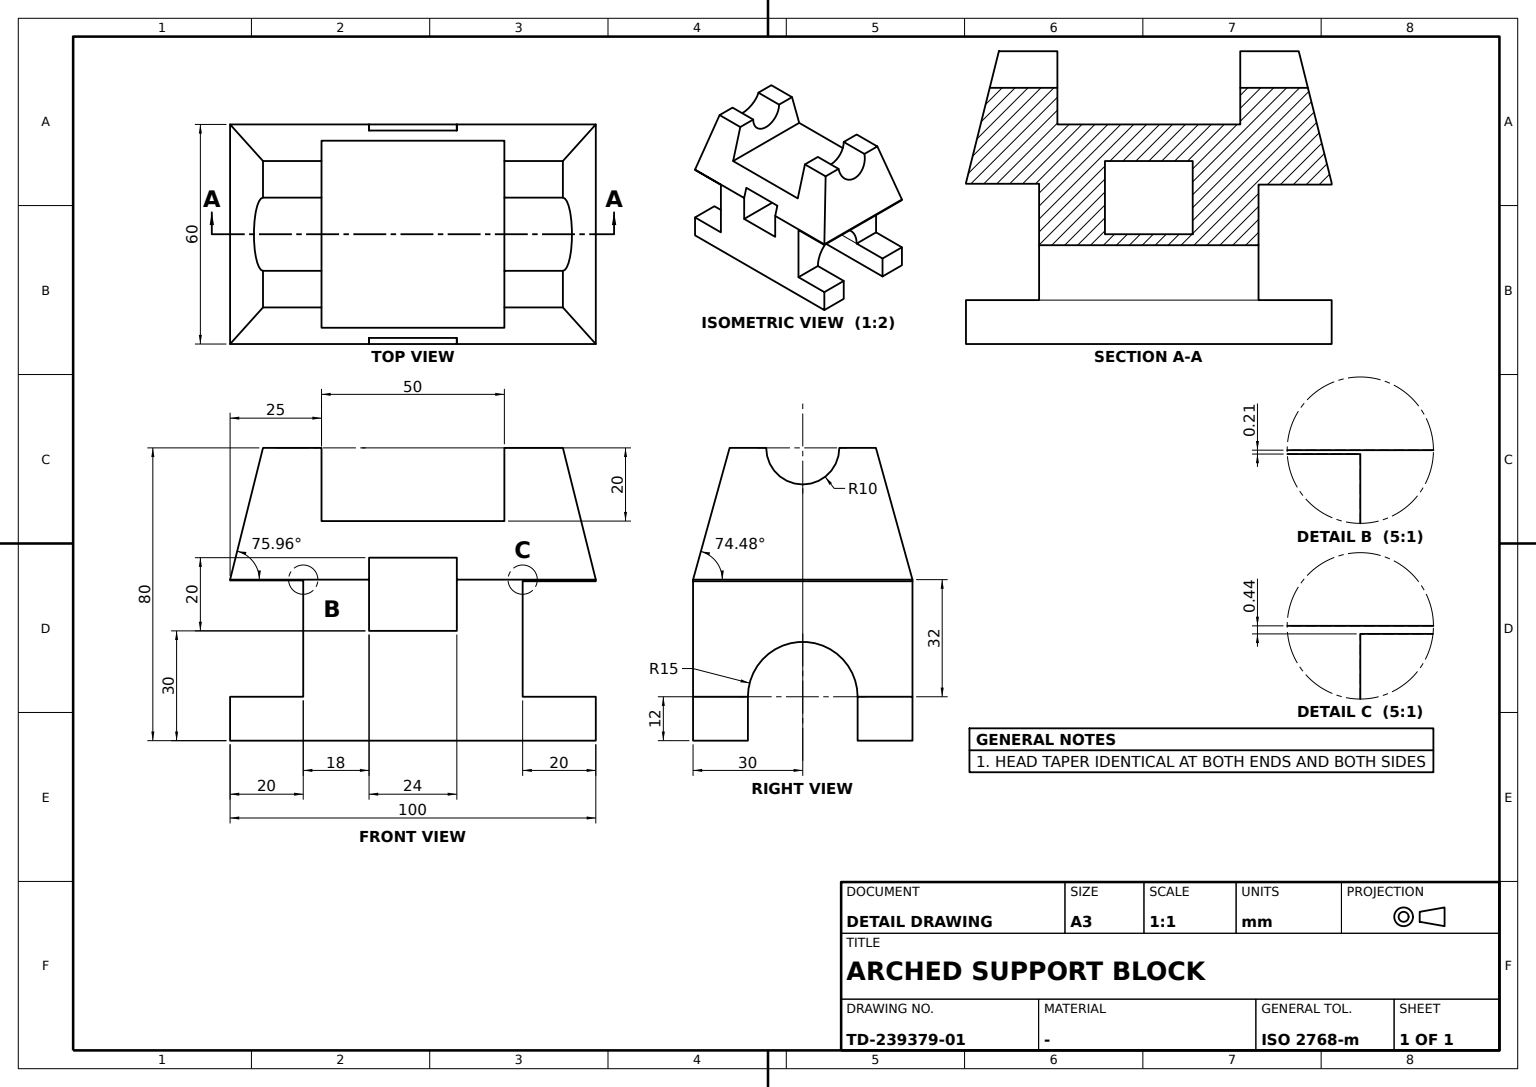
ISO-10303-21;
HEADER;
FILE_DESCRIPTION((''),'2;1');
FILE_NAME('','',(''),(''),'','','');
FILE_SCHEMA(('AUTOMOTIVE_DESIGN'));
ENDSEC;
DATA;
#1=APPLICATION_CONTEXT('');
#2=PRODUCT_CONTEXT('',#1,'mechanical');
#3=PRODUCT('','','',(#2));
#4=PRODUCT_DEFINITION_FORMATION('','',#3);
#5=PRODUCT_DEFINITION_CONTEXT('',#1,'design');
#6=PRODUCT_DEFINITION('','',#4,#5);
#7=PRODUCT_DEFINITION_SHAPE('','',#6);
#8=(LENGTH_UNIT()NAMED_UNIT(*)SI_UNIT(.MILLI.,.METRE.));
#9=(NAMED_UNIT(*)PLANE_ANGLE_UNIT()SI_UNIT($,.RADIAN.));
#10=(NAMED_UNIT(*)SI_UNIT($,.STERADIAN.)SOLID_ANGLE_UNIT());
#11=UNCERTAINTY_MEASURE_WITH_UNIT(LENGTH_MEASURE(0.005),#8,'distance_accuracy_value','');
#12=(GEOMETRIC_REPRESENTATION_CONTEXT(3)GLOBAL_UNCERTAINTY_ASSIGNED_CONTEXT((#11))GLOBAL_UNIT_ASSIGNED_CONTEXT((#8,#9,#10))REPRESENTATION_CONTEXT('',''));
#13=CARTESIAN_POINT('',(40.,25.,80.));
#14=VERTEX_POINT('',#13);
#15=CARTESIAN_POINT('',(20.,25.,80.));
#16=VERTEX_POINT('',#15);
#17=CARTESIAN_POINT('',(30.,25.,80.));
#18=DIRECTION('',(0.,1.,0.));
#19=DIRECTION('',(0.,0.,1.));
#20=AXIS2_PLACEMENT_3D('',#17,#18,#19);
#21=CIRCLE('',#20,10.);
#22=EDGE_CURVE('',#14,#16,#21,.T.);
#23=ORIENTED_EDGE('',*,*,#22,.T.);
#24=CARTESIAN_POINT('',(20.,9.,80.));
#25=VERTEX_POINT('',#24);
#26=VECTOR('',#18,1000.);
#27=LINE('',#24,#26);
#28=EDGE_CURVE('',#25,#16,#27,.T.);
#29=ORIENTED_EDGE('',*,*,#28,.F.);
#30=CARTESIAN_POINT('',(40.,9.,80.));
#31=VERTEX_POINT('',#30);
#32=CARTESIAN_POINT('',(30.,9.,80.));
#33=DIRECTION('',(0.,-0.9701425,0.242535625));
#34=DIRECTION('',(0.,0.242535625,0.9701425));
#35=AXIS2_PLACEMENT_3D('',#32,#33,#34);
#36=ELLIPSE('',#35,10.307764,10.);
#37=EDGE_CURVE('',#25,#31,#36,.T.);
#38=ORIENTED_EDGE('',*,*,#37,.T.);
#39=LINE('',#30,#26);
#40=EDGE_CURVE('',#14,#31,#39,.F.);
#41=ORIENTED_EDGE('',*,*,#40,.F.);
#42=EDGE_LOOP('',(#23,#29,#38,#41));
#43=FACE_BOUND('',#42,.T.);
#44=CARTESIAN_POINT('',(30.,49.34,80.));
#45=DIRECTION('',(-1.,0.,0.));
#46=AXIS2_PLACEMENT_3D('',#44,#18,#45);
#47=CYLINDRICAL_SURFACE('',#46,10.);
#48=ADVANCED_FACE('',(#43),#47,.F.);
#49=CARTESIAN_POINT('',(60.,100.,0.));
#50=VERTEX_POINT('',#49);
#51=CARTESIAN_POINT('',(60.,100.,12.));
#52=VERTEX_POINT('',#51);
#53=VECTOR('',#19,1000.);
#54=LINE('',#49,#53);
#55=EDGE_CURVE('',#50,#52,#54,.T.);
#56=ORIENTED_EDGE('',*,*,#55,.F.);
#57=CARTESIAN_POINT('',(45.,100.,0.));
#58=VERTEX_POINT('',#57);
#59=CARTESIAN_POINT('',(0.,100.,0.));
#60=VECTOR('',#45,1000.);
#61=LINE('',#59,#60);
#62=EDGE_CURVE('',#50,#58,#61,.T.);
#63=ORIENTED_EDGE('',*,*,#62,.T.);
#64=CARTESIAN_POINT('',(45.,100.,12.));
#65=VERTEX_POINT('',#64);
#66=DIRECTION('',(0.,0.,-1.));
#67=VECTOR('',#66,1000.);
#68=LINE('',#64,#67);
#69=EDGE_CURVE('',#65,#58,#68,.T.);
#70=ORIENTED_EDGE('',*,*,#69,.F.);
#71=CARTESIAN_POINT('',(15.,100.,12.));
#72=LINE('',#71,#60);
#73=EDGE_CURVE('',#52,#65,#72,.T.);
#74=ORIENTED_EDGE('',*,*,#73,.F.);
#75=EDGE_LOOP('',(#56,#63,#70,#74));
#76=FACE_BOUND('',#75,.T.);
#77=AXIS2_PLACEMENT_3D('',#49,#18,#45);
#78=PLANE('',#77);
#79=ADVANCED_FACE('',(#76),#78,.T.);
#80=CARTESIAN_POINT('',(60.,0.,0.));
#81=VERTEX_POINT('',#80);
#82=CARTESIAN_POINT('',(60.,0.,12.));
#83=VERTEX_POINT('',#82);
#84=LINE('',#80,#53);
#85=EDGE_CURVE('',#81,#83,#84,.T.);
#86=ORIENTED_EDGE('',*,*,#85,.T.);
#87=CARTESIAN_POINT('',(45.,0.,12.));
#88=VERTEX_POINT('',#87);
#89=CARTESIAN_POINT('',(15.,0.,12.));
#90=DIRECTION('',(1.,0.,0.));
#91=VECTOR('',#90,1000.);
#92=LINE('',#89,#91);
#93=EDGE_CURVE('',#88,#83,#92,.T.);
#94=ORIENTED_EDGE('',*,*,#93,.F.);
#95=CARTESIAN_POINT('',(45.,0.,0.));
#96=VERTEX_POINT('',#95);
#97=LINE('',#95,#67);
#98=EDGE_CURVE('',#88,#96,#97,.T.);
#99=ORIENTED_EDGE('',*,*,#98,.T.);
#100=CARTESIAN_POINT('',(0.,0.,0.));
#101=LINE('',#100,#91);
#102=EDGE_CURVE('',#96,#81,#101,.T.);
#103=ORIENTED_EDGE('',*,*,#102,.T.);
#104=EDGE_LOOP('',(#86,#94,#99,#103));
#105=FACE_BOUND('',#104,.T.);
#106=DIRECTION('',(0.,-1.,0.));
#107=AXIS2_PLACEMENT_3D('',#100,#106,#90);
#108=PLANE('',#107);
#109=ADVANCED_FACE('',(#105),#108,.T.);
#110=CARTESIAN_POINT('',(15.,80.,12.));
#111=VERTEX_POINT('',#110);
#112=CARTESIAN_POINT('',(0.,80.,12.));
#113=VERTEX_POINT('',#112);
#114=LINE('',#110,#60);
#115=EDGE_CURVE('',#111,#113,#114,.T.);
#116=ORIENTED_EDGE('',*,*,#115,.T.);
#117=CARTESIAN_POINT('',(0.,80.,43.56));
#118=VERTEX_POINT('',#117);
#119=CARTESIAN_POINT('',(0.,80.,0.));
#120=LINE('',#119,#53);
#121=EDGE_CURVE('',#113,#118,#120,.T.);
#122=ORIENTED_EDGE('',*,*,#121,.T.);
#123=CARTESIAN_POINT('',(60.,80.,43.56));
#124=VERTEX_POINT('',#123);
#125=LINE('',#117,#91);
#126=EDGE_CURVE('',#118,#124,#125,.T.);
#127=ORIENTED_EDGE('',*,*,#126,.T.);
#128=CARTESIAN_POINT('',(60.,80.,12.));
#129=VERTEX_POINT('',#128);
#130=CARTESIAN_POINT('',(60.,80.,0.));
#131=LINE('',#130,#67);
#132=EDGE_CURVE('',#124,#129,#131,.T.);
#133=ORIENTED_EDGE('',*,*,#132,.T.);
#134=CARTESIAN_POINT('',(45.,80.,12.));
#135=VERTEX_POINT('',#134);
#136=EDGE_CURVE('',#129,#135,#114,.T.);
#137=ORIENTED_EDGE('',*,*,#136,.T.);
#138=CARTESIAN_POINT('',(30.,80.,12.));
#139=AXIS2_PLACEMENT_3D('',#138,#18,#19);
#140=CIRCLE('',#139,15.);
#141=EDGE_CURVE('',#111,#135,#140,.T.);
#142=ORIENTED_EDGE('',*,*,#141,.F.);
#143=EDGE_LOOP('',(#116,#122,#127,#133,#137,#142));
#144=FACE_BOUND('',#143,.T.);
#145=AXIS2_PLACEMENT_3D('',#119,#18,#45);
#146=PLANE('',#145);
#147=ADVANCED_FACE('',(#144),#146,.T.);
#148=CARTESIAN_POINT('',(1.666667,38.,50.));
#149=VERTEX_POINT('',#148);
#150=CARTESIAN_POINT('',(58.333333,38.,50.));
#151=VERTEX_POINT('',#150);
#152=CARTESIAN_POINT('',(0.,38.,50.));
#153=LINE('',#152,#91);
#154=EDGE_CURVE('',#149,#151,#153,.T.);
#155=ORIENTED_EDGE('',*,*,#154,.T.);
#156=CARTESIAN_POINT('',(60.,38.,44.));
#157=VERTEX_POINT('',#156);
#158=CARTESIAN_POINT('',(59.312321,38.,46.475645));
#159=DIRECTION('',(0.267643864,0.,-0.96351791));
#160=VECTOR('',#159,1000.);
#161=LINE('',#158,#160);
#162=EDGE_CURVE('',#151,#157,#161,.T.);
#163=ORIENTED_EDGE('',*,*,#162,.T.);
#164=CARTESIAN_POINT('',(60.,38.,30.));
#165=VERTEX_POINT('',#164);
#166=LINE('',#164,#53);
#167=EDGE_CURVE('',#165,#157,#166,.T.);
#168=ORIENTED_EDGE('',*,*,#167,.F.);
#169=CARTESIAN_POINT('',(0.,38.,30.));
#170=VERTEX_POINT('',#169);
#171=LINE('',#169,#91);
#172=EDGE_CURVE('',#170,#165,#171,.T.);
#173=ORIENTED_EDGE('',*,*,#172,.F.);
#174=CARTESIAN_POINT('',(0.,38.,44.));
#175=VERTEX_POINT('',#174);
#176=CARTESIAN_POINT('',(0.,38.,0.));
#177=LINE('',#176,#53);
#178=EDGE_CURVE('',#170,#175,#177,.T.);
#179=ORIENTED_EDGE('',*,*,#178,.T.);
#180=DIRECTION('',(0.267643864,0.,0.96351791));
#181=VECTOR('',#180,1000.);
#182=LINE('',#174,#181);
#183=EDGE_CURVE('',#175,#149,#182,.T.);
#184=ORIENTED_EDGE('',*,*,#183,.T.);
#185=EDGE_LOOP('',(#155,#163,#168,#173,#179,#184));
#186=FACE_BOUND('',#185,.T.);
#187=AXIS2_PLACEMENT_3D('',#169,#18,#19);
#188=PLANE('',#187);
#189=ADVANCED_FACE('',(#186),#188,.T.);
#190=VERTEX_POINT('',#100);
#191=CARTESIAN_POINT('',(0.,0.,12.));
#192=VERTEX_POINT('',#191);
#193=LINE('',#100,#53);
#194=EDGE_CURVE('',#190,#192,#193,.T.);
#195=ORIENTED_EDGE('',*,*,#194,.F.);
#196=CARTESIAN_POINT('',(15.,0.,0.));
#197=VERTEX_POINT('',#196);
#198=EDGE_CURVE('',#190,#197,#101,.T.);
#199=ORIENTED_EDGE('',*,*,#198,.T.);
#200=VERTEX_POINT('',#89);
#201=LINE('',#196,#53);
#202=EDGE_CURVE('',#197,#200,#201,.T.);
#203=ORIENTED_EDGE('',*,*,#202,.T.);
#204=EDGE_CURVE('',#192,#200,#92,.T.);
#205=ORIENTED_EDGE('',*,*,#204,.F.);
#206=EDGE_LOOP('',(#195,#199,#203,#205));
#207=FACE_BOUND('',#206,.T.);
#208=ADVANCED_FACE('',(#207),#108,.T.);
#209=CARTESIAN_POINT('',(0.,62.,30.));
#210=VERTEX_POINT('',#209);
#211=CARTESIAN_POINT('',(60.,62.,30.));
#212=VERTEX_POINT('',#211);
#213=LINE('',#209,#91);
#214=EDGE_CURVE('',#210,#212,#213,.T.);
#215=ORIENTED_EDGE('',*,*,#214,.F.);
#216=CARTESIAN_POINT('',(0.,0.,30.));
#217=LINE('',#216,#26);
#218=EDGE_CURVE('',#170,#210,#217,.T.);
#219=ORIENTED_EDGE('',*,*,#218,.F.);
#220=ORIENTED_EDGE('',*,*,#172,.T.);
#221=LINE('',#164,#26);
#222=EDGE_CURVE('',#165,#212,#221,.T.);
#223=ORIENTED_EDGE('',*,*,#222,.T.);
#224=EDGE_LOOP('',(#215,#219,#220,#223));
#225=FACE_BOUND('',#224,.T.);
#226=AXIS2_PLACEMENT_3D('',#169,#66,#18);
#227=PLANE('',#226);
#228=ADVANCED_FACE('',(#225),#227,.F.);
#229=CARTESIAN_POINT('',(40.,91.,80.));
#230=VERTEX_POINT('',#229);
#231=CARTESIAN_POINT('',(50.,91.,80.));
#232=VERTEX_POINT('',#231);
#233=LINE('',#231,#91);
#234=EDGE_CURVE('',#230,#232,#233,.T.);
#235=ORIENTED_EDGE('',*,*,#234,.F.);
#236=CARTESIAN_POINT('',(40.,75.,80.));
#237=VERTEX_POINT('',#236);
#238=LINE('',#236,#26);
#239=EDGE_CURVE('',#230,#237,#238,.F.);
#240=ORIENTED_EDGE('',*,*,#239,.T.);
#241=CARTESIAN_POINT('',(50.,75.,80.));
#242=VERTEX_POINT('',#241);
#243=LINE('',#241,#91);
#244=EDGE_CURVE('',#237,#242,#243,.T.);
#245=ORIENTED_EDGE('',*,*,#244,.T.);
#246=CARTESIAN_POINT('',(50.,100.,80.));
#247=VECTOR('',#106,1000.);
#248=LINE('',#246,#247);
#249=EDGE_CURVE('',#232,#242,#248,.T.);
#250=ORIENTED_EDGE('',*,*,#249,.F.);
#251=EDGE_LOOP('',(#235,#240,#245,#250));
#252=FACE_BOUND('',#251,.T.);
#253=AXIS2_PLACEMENT_3D('',#246,#19,#45);
#254=PLANE('',#253);
#255=ADVANCED_FACE('',(#252),#254,.T.);
#256=CARTESIAN_POINT('',(0.,100.,44.));
#257=VERTEX_POINT('',#256);
#258=CARTESIAN_POINT('',(60.,100.,44.));
#259=VERTEX_POINT('',#258);
#260=LINE('',#256,#91);
#261=EDGE_CURVE('',#257,#259,#260,.T.);
#262=ORIENTED_EDGE('',*,*,#261,.F.);
#263=CARTESIAN_POINT('',(10.,91.,80.));
#264=VERTEX_POINT('',#263);
#265=CARTESIAN_POINT('',(9.322952,91.609343,77.562627));
#266=DIRECTION('',(0.260201474,-0.234181327,0.936725306));
#267=VECTOR('',#266,1000.);
#268=LINE('',#265,#267);
#269=EDGE_CURVE('',#257,#264,#268,.T.);
#270=ORIENTED_EDGE('',*,*,#269,.T.);
#271=CARTESIAN_POINT('',(20.,91.,80.));
#272=VERTEX_POINT('',#271);
#273=EDGE_CURVE('',#264,#272,#233,.T.);
#274=ORIENTED_EDGE('',*,*,#273,.T.);
#275=CARTESIAN_POINT('',(30.,91.,80.));
#276=DIRECTION('',(0.,-0.9701425,-0.242535625));
#277=DIRECTION('',(0.,0.242535625,-0.9701425));
#278=AXIS2_PLACEMENT_3D('',#275,#276,#277);
#279=ELLIPSE('',#278,10.307764,10.);
#280=EDGE_CURVE('',#272,#230,#279,.T.);
#281=ORIENTED_EDGE('',*,*,#280,.T.);
#282=ORIENTED_EDGE('',*,*,#234,.T.);
#283=CARTESIAN_POINT('',(46.61476,87.953284,92.186865));
#284=DIRECTION('',(-0.260201474,-0.234181327,0.936725306));
#285=VECTOR('',#284,1000.);
#286=LINE('',#283,#285);
#287=EDGE_CURVE('',#259,#232,#286,.T.);
#288=ORIENTED_EDGE('',*,*,#287,.F.);
#289=EDGE_LOOP('',(#262,#270,#274,#281,#282,#288));
#290=FACE_BOUND('',#289,.T.);
#291=CARTESIAN_POINT('',(0.,91.,80.));
#292=AXIS2_PLACEMENT_3D('',#291,#276,#277);
#293=PLANE('',#292);
#294=ADVANCED_FACE('',(#290),#293,.F.);
#295=CARTESIAN_POINT('',(50.,25.,80.));
#296=VERTEX_POINT('',#295);
#297=CARTESIAN_POINT('',(55.555556,25.,60.));
#298=VERTEX_POINT('',#297);
#299=CARTESIAN_POINT('',(51.575931,25.,74.326648));
#300=LINE('',#299,#160);
#301=EDGE_CURVE('',#296,#298,#300,.T.);
#302=ORIENTED_EDGE('',*,*,#301,.T.);
#303=CARTESIAN_POINT('',(4.444444,25.,60.));
#304=VERTEX_POINT('',#303);
#305=CARTESIAN_POINT('',(0.,25.,60.));
#306=LINE('',#305,#91);
#307=EDGE_CURVE('',#304,#298,#306,.T.);
#308=ORIENTED_EDGE('',*,*,#307,.F.);
#309=CARTESIAN_POINT('',(10.,25.,80.));
#310=VERTEX_POINT('',#309);
#311=CARTESIAN_POINT('',(4.126074,25.,58.853868));
#312=DIRECTION('',(-0.267643864,0.,-0.96351791));
#313=VECTOR('',#312,1000.);
#314=LINE('',#311,#313);
#315=EDGE_CURVE('',#310,#304,#314,.T.);
#316=ORIENTED_EDGE('',*,*,#315,.F.);
#317=CARTESIAN_POINT('',(0.,25.,80.));
#318=LINE('',#317,#91);
#319=EDGE_CURVE('',#310,#16,#318,.T.);
#320=ORIENTED_EDGE('',*,*,#319,.T.);
#321=ORIENTED_EDGE('',*,*,#22,.F.);
#322=EDGE_CURVE('',#14,#296,#318,.T.);
#323=ORIENTED_EDGE('',*,*,#322,.T.);
#324=EDGE_LOOP('',(#302,#308,#316,#320,#321,#323));
#325=FACE_BOUND('',#324,.T.);
#326=AXIS2_PLACEMENT_3D('',#305,#18,#19);
#327=PLANE('',#326);
#328=ADVANCED_FACE('',(#325),#327,.T.);
#329=CARTESIAN_POINT('',(0.,20.,12.));
#330=VERTEX_POINT('',#329);
#331=CARTESIAN_POINT('',(15.,20.,12.));
#332=VERTEX_POINT('',#331);
#333=LINE('',#331,#91);
#334=EDGE_CURVE('',#330,#332,#333,.T.);
#335=ORIENTED_EDGE('',*,*,#334,.T.);
#336=CARTESIAN_POINT('',(45.,20.,12.));
#337=VERTEX_POINT('',#336);
#338=CARTESIAN_POINT('',(30.,20.,12.));
#339=AXIS2_PLACEMENT_3D('',#338,#106,#66);
#340=CIRCLE('',#339,15.);
#341=EDGE_CURVE('',#337,#332,#340,.T.);
#342=ORIENTED_EDGE('',*,*,#341,.F.);
#343=CARTESIAN_POINT('',(60.,20.,12.));
#344=VERTEX_POINT('',#343);
#345=EDGE_CURVE('',#337,#344,#333,.T.);
#346=ORIENTED_EDGE('',*,*,#345,.T.);
#347=CARTESIAN_POINT('',(60.,20.,43.788128));
#348=VERTEX_POINT('',#347);
#349=CARTESIAN_POINT('',(60.,20.,0.));
#350=LINE('',#349,#53);
#351=EDGE_CURVE('',#344,#348,#350,.T.);
#352=ORIENTED_EDGE('',*,*,#351,.T.);
#353=CARTESIAN_POINT('',(0.,20.,43.788128));
#354=VERTEX_POINT('',#353);
#355=LINE('',#347,#60);
#356=EDGE_CURVE('',#348,#354,#355,.T.);
#357=ORIENTED_EDGE('',*,*,#356,.T.);
#358=CARTESIAN_POINT('',(0.,20.,0.));
#359=LINE('',#358,#67);
#360=EDGE_CURVE('',#354,#330,#359,.T.);
#361=ORIENTED_EDGE('',*,*,#360,.T.);
#362=EDGE_LOOP('',(#335,#342,#346,#352,#357,#361));
#363=FACE_BOUND('',#362,.T.);
#364=AXIS2_PLACEMENT_3D('',#358,#106,#90);
#365=PLANE('',#364);
#366=ADVANCED_FACE('',(#363),#365,.T.);
#367=LINE('',#95,#247);
#368=EDGE_CURVE('',#58,#96,#367,.T.);
#369=ORIENTED_EDGE('',*,*,#368,.T.);
#370=ORIENTED_EDGE('',*,*,#98,.F.);
#371=LINE('',#64,#26);
#372=EDGE_CURVE('',#88,#337,#371,.T.);
#373=ORIENTED_EDGE('',*,*,#372,.T.);
#374=CARTESIAN_POINT('',(45.,50.,12.));
#375=LINE('',#374,#26);
#376=EDGE_CURVE('',#135,#337,#375,.F.);
#377=ORIENTED_EDGE('',*,*,#376,.F.);
#378=LINE('',#64,#247);
#379=EDGE_CURVE('',#65,#135,#378,.T.);
#380=ORIENTED_EDGE('',*,*,#379,.F.);
#381=ORIENTED_EDGE('',*,*,#69,.T.);
#382=EDGE_LOOP('',(#369,#370,#373,#377,#380,#381));
#383=FACE_BOUND('',#382,.T.);
#384=AXIS2_PLACEMENT_3D('',#64,#45,#66);
#385=PLANE('',#384);
#386=ADVANCED_FACE('',(#383),#385,.T.);
#387=CARTESIAN_POINT('',(55.555556,75.,60.));
#388=VERTEX_POINT('',#387);
#389=CARTESIAN_POINT('',(55.555556,100.,60.));
#390=LINE('',#389,#26);
#391=EDGE_CURVE('',#298,#388,#390,.T.);
#392=ORIENTED_EDGE('',*,*,#391,.T.);
#393=CARTESIAN_POINT('',(4.444444,75.,60.));
#394=VERTEX_POINT('',#393);
#395=CARTESIAN_POINT('',(0.,75.,60.));
#396=LINE('',#395,#91);
#397=EDGE_CURVE('',#394,#388,#396,.T.);
#398=ORIENTED_EDGE('',*,*,#397,.F.);
#399=CARTESIAN_POINT('',(4.444444,100.,60.));
#400=LINE('',#399,#26);
#401=EDGE_CURVE('',#304,#394,#400,.T.);
#402=ORIENTED_EDGE('',*,*,#401,.F.);
#403=ORIENTED_EDGE('',*,*,#307,.T.);
#404=EDGE_LOOP('',(#392,#398,#402,#403));
#405=FACE_BOUND('',#404,.T.);
#406=AXIS2_PLACEMENT_3D('',#305,#66,#18);
#407=PLANE('',#406);
#408=ADVANCED_FACE('',(#405),#407,.F.);
#409=ORIENTED_EDGE('',*,*,#368,.F.);
#410=ORIENTED_EDGE('',*,*,#62,.F.);
#411=LINE('',#80,#247);
#412=EDGE_CURVE('',#50,#81,#411,.T.);
#413=ORIENTED_EDGE('',*,*,#412,.T.);
#414=ORIENTED_EDGE('',*,*,#102,.F.);
#415=EDGE_LOOP('',(#409,#410,#413,#414));
#416=FACE_BOUND('',#415,.T.);
#417=AXIS2_PLACEMENT_3D('',#100,#19,#18);
#418=PLANE('',#417);
#419=ADVANCED_FACE('',(#416),#418,.F.);
#420=ORIENTED_EDGE('',*,*,#249,.T.);
#421=CARTESIAN_POINT('',(60.,75.,44.));
#422=LINE('',#421,#160);
#423=EDGE_CURVE('',#242,#388,#422,.T.);
#424=ORIENTED_EDGE('',*,*,#423,.T.);
#425=ORIENTED_EDGE('',*,*,#391,.F.);
#426=ORIENTED_EDGE('',*,*,#301,.F.);
#427=CARTESIAN_POINT('',(50.,9.,80.));
#428=VERTEX_POINT('',#427);
#429=EDGE_CURVE('',#296,#428,#248,.T.);
#430=ORIENTED_EDGE('',*,*,#429,.T.);
#431=CARTESIAN_POINT('',(60.,0.,44.));
#432=VERTEX_POINT('',#431);
#433=CARTESIAN_POINT('',(46.61476,12.046716,92.186865));
#434=DIRECTION('',(-0.260201474,0.234181327,0.936725306));
#435=VECTOR('',#434,1000.);
#436=LINE('',#433,#435);
#437=EDGE_CURVE('',#432,#428,#436,.T.);
#438=ORIENTED_EDGE('',*,*,#437,.F.);
#439=LINE('',#258,#247);
#440=EDGE_CURVE('',#157,#432,#439,.T.);
#441=ORIENTED_EDGE('',*,*,#440,.F.);
#442=ORIENTED_EDGE('',*,*,#162,.F.);
#443=CARTESIAN_POINT('',(58.333333,62.,50.));
#444=VERTEX_POINT('',#443);
#445=CARTESIAN_POINT('',(58.333333,100.,50.));
#446=LINE('',#445,#247);
#447=EDGE_CURVE('',#444,#151,#446,.T.);
#448=ORIENTED_EDGE('',*,*,#447,.F.);
#449=CARTESIAN_POINT('',(60.,62.,44.));
#450=VERTEX_POINT('',#449);
#451=LINE('',#449,#160);
#452=EDGE_CURVE('',#444,#450,#451,.T.);
#453=ORIENTED_EDGE('',*,*,#452,.T.);
#454=EDGE_CURVE('',#259,#450,#439,.T.);
#455=ORIENTED_EDGE('',*,*,#454,.F.);
#456=ORIENTED_EDGE('',*,*,#287,.T.);
#457=EDGE_LOOP('',(#420,#424,#425,#426,#430,#438,#441,#442,#448,#453,#455,#456));
#458=FACE_BOUND('',#457,.T.);
#459=DIRECTION('',(0.96351791,0.,0.267643864));
#460=DIRECTION('',(-0.267643864,0.,0.96351791));
#461=AXIS2_PLACEMENT_3D('',#258,#459,#460);
#462=PLANE('',#461);
#463=ADVANCED_FACE('',(#458),#462,.T.);
#464=ORIENTED_EDGE('',*,*,#204,.T.);
#465=LINE('',#71,#26);
#466=EDGE_CURVE('',#200,#332,#465,.T.);
#467=ORIENTED_EDGE('',*,*,#466,.T.);
#468=ORIENTED_EDGE('',*,*,#334,.F.);
#469=CARTESIAN_POINT('',(0.,100.,12.));
#470=LINE('',#469,#26);
#471=EDGE_CURVE('',#192,#330,#470,.T.);
#472=ORIENTED_EDGE('',*,*,#471,.F.);
#473=EDGE_LOOP('',(#464,#467,#468,#472));
#474=FACE_BOUND('',#473,.T.);
#475=AXIS2_PLACEMENT_3D('',#71,#19,#45);
#476=PLANE('',#475);
#477=ADVANCED_FACE('',(#474),#476,.T.);
#478=CARTESIAN_POINT('',(60.,62.,0.));
#479=LINE('',#478,#53);
#480=EDGE_CURVE('',#212,#450,#479,.T.);
#481=ORIENTED_EDGE('',*,*,#480,.T.);
#482=ORIENTED_EDGE('',*,*,#452,.F.);
#483=CARTESIAN_POINT('',(1.666667,62.,50.));
#484=VERTEX_POINT('',#483);
#485=CARTESIAN_POINT('',(0.,62.,50.));
#486=LINE('',#485,#91);
#487=EDGE_CURVE('',#484,#444,#486,.T.);
#488=ORIENTED_EDGE('',*,*,#487,.F.);
#489=CARTESIAN_POINT('',(0.,62.,44.));
#490=VERTEX_POINT('',#489);
#491=CARTESIAN_POINT('',(1.547278,62.,49.570201));
#492=LINE('',#491,#181);
#493=EDGE_CURVE('',#490,#484,#492,.T.);
#494=ORIENTED_EDGE('',*,*,#493,.F.);
#495=CARTESIAN_POINT('',(0.,62.,0.));
#496=LINE('',#495,#67);
#497=EDGE_CURVE('',#490,#210,#496,.T.);
#498=ORIENTED_EDGE('',*,*,#497,.T.);
#499=ORIENTED_EDGE('',*,*,#214,.T.);
#500=EDGE_LOOP('',(#481,#482,#488,#494,#498,#499));
#501=FACE_BOUND('',#500,.T.);
#502=AXIS2_PLACEMENT_3D('',#485,#106,#66);
#503=PLANE('',#502);
#504=ADVANCED_FACE('',(#501),#503,.T.);
#505=CARTESIAN_POINT('',(15.,50.,12.));
#506=LINE('',#505,#26);
#507=EDGE_CURVE('',#111,#332,#506,.F.);
#508=ORIENTED_EDGE('',*,*,#507,.F.);
#509=ORIENTED_EDGE('',*,*,#141,.T.);
#510=ORIENTED_EDGE('',*,*,#376,.T.);
#511=ORIENTED_EDGE('',*,*,#341,.T.);
#512=EDGE_LOOP('',(#508,#509,#510,#511));
#513=FACE_BOUND('',#512,.T.);
#514=CARTESIAN_POINT('',(30.,50.,12.));
#515=AXIS2_PLACEMENT_3D('',#514,#18,#45);
#516=CYLINDRICAL_SURFACE('',#515,15.);
#517=ADVANCED_FACE('',(#513),#516,.F.);
#518=CARTESIAN_POINT('',(0.,0.,44.));
#519=VERTEX_POINT('',#518);
#520=LINE('',#518,#91);
#521=EDGE_CURVE('',#519,#432,#520,.T.);
#522=ORIENTED_EDGE('',*,*,#521,.T.);
#523=ORIENTED_EDGE('',*,*,#437,.T.);
#524=LINE('',#427,#91);
#525=EDGE_CURVE('',#31,#428,#524,.T.);
#526=ORIENTED_EDGE('',*,*,#525,.F.);
#527=ORIENTED_EDGE('',*,*,#37,.F.);
#528=CARTESIAN_POINT('',(10.,9.,80.));
#529=VERTEX_POINT('',#528);
#530=EDGE_CURVE('',#529,#25,#524,.T.);
#531=ORIENTED_EDGE('',*,*,#530,.F.);
#532=CARTESIAN_POINT('',(9.322952,8.390657,77.562627));
#533=DIRECTION('',(0.260201474,0.234181327,0.936725306));
#534=VECTOR('',#533,1000.);
#535=LINE('',#532,#534);
#536=EDGE_CURVE('',#519,#529,#535,.T.);
#537=ORIENTED_EDGE('',*,*,#536,.F.);
#538=EDGE_LOOP('',(#522,#523,#526,#527,#531,#537));
#539=FACE_BOUND('',#538,.T.);
#540=CARTESIAN_POINT('',(0.,9.,80.));
#541=DIRECTION('',(0.,-0.242535625,-0.9701425));
#542=AXIS2_PLACEMENT_3D('',#540,#33,#541);
#543=PLANE('',#542);
#544=ADVANCED_FACE('',(#539),#543,.T.);
#545=VERTEX_POINT('',#59);
#546=VERTEX_POINT('',#469);
#547=LINE('',#59,#53);
#548=EDGE_CURVE('',#545,#546,#547,.T.);
#549=ORIENTED_EDGE('',*,*,#548,.T.);
#550=VERTEX_POINT('',#71);
#551=EDGE_CURVE('',#550,#546,#72,.T.);
#552=ORIENTED_EDGE('',*,*,#551,.F.);
#553=CARTESIAN_POINT('',(15.,100.,0.));
#554=VERTEX_POINT('',#553);
#555=LINE('',#553,#53);
#556=EDGE_CURVE('',#554,#550,#555,.T.);
#557=ORIENTED_EDGE('',*,*,#556,.F.);
#558=EDGE_CURVE('',#554,#545,#61,.T.);
#559=ORIENTED_EDGE('',*,*,#558,.T.);
#560=EDGE_LOOP('',(#549,#552,#557,#559));
#561=FACE_BOUND('',#560,.T.);
#562=ADVANCED_FACE('',(#561),#78,.T.);
#563=ORIENTED_EDGE('',*,*,#73,.T.);
#564=ORIENTED_EDGE('',*,*,#379,.T.);
#565=ORIENTED_EDGE('',*,*,#136,.F.);
#566=LINE('',#51,#247);
#567=EDGE_CURVE('',#52,#129,#566,.T.);
#568=ORIENTED_EDGE('',*,*,#567,.F.);
#569=EDGE_LOOP('',(#563,#564,#565,#568));
#570=FACE_BOUND('',#569,.T.);
#571=ADVANCED_FACE('',(#570),#476,.T.);
#572=CARTESIAN_POINT('',(10.,75.,80.));
#573=VERTEX_POINT('',#572);
#574=CARTESIAN_POINT('',(20.,75.,80.));
#575=VERTEX_POINT('',#574);
#576=EDGE_CURVE('',#573,#575,#243,.T.);
#577=ORIENTED_EDGE('',*,*,#576,.T.);
#578=LINE('',#574,#26);
#579=EDGE_CURVE('',#575,#272,#578,.T.);
#580=ORIENTED_EDGE('',*,*,#579,.T.);
#581=ORIENTED_EDGE('',*,*,#273,.F.);
#582=CARTESIAN_POINT('',(10.,100.,80.));
#583=LINE('',#582,#247);
#584=EDGE_CURVE('',#264,#573,#583,.T.);
#585=ORIENTED_EDGE('',*,*,#584,.T.);
#586=EDGE_LOOP('',(#577,#580,#581,#585));
#587=FACE_BOUND('',#586,.T.);
#588=ADVANCED_FACE('',(#587),#254,.T.);
#589=ORIENTED_EDGE('',*,*,#315,.T.);
#590=ORIENTED_EDGE('',*,*,#401,.T.);
#591=CARTESIAN_POINT('',(0.,75.,44.));
#592=LINE('',#591,#313);
#593=EDGE_CURVE('',#573,#394,#592,.T.);
#594=ORIENTED_EDGE('',*,*,#593,.F.);
#595=ORIENTED_EDGE('',*,*,#584,.F.);
#596=ORIENTED_EDGE('',*,*,#269,.F.);
#597=LINE('',#256,#247);
#598=EDGE_CURVE('',#257,#490,#597,.T.);
#599=ORIENTED_EDGE('',*,*,#598,.T.);
#600=ORIENTED_EDGE('',*,*,#493,.T.);
#601=CARTESIAN_POINT('',(1.666667,100.,50.));
#602=LINE('',#601,#247);
#603=EDGE_CURVE('',#484,#149,#602,.T.);
#604=ORIENTED_EDGE('',*,*,#603,.T.);
#605=ORIENTED_EDGE('',*,*,#183,.F.);
#606=EDGE_CURVE('',#175,#519,#597,.T.);
#607=ORIENTED_EDGE('',*,*,#606,.T.);
#608=ORIENTED_EDGE('',*,*,#536,.T.);
#609=EDGE_CURVE('',#310,#529,#583,.T.);
#610=ORIENTED_EDGE('',*,*,#609,.F.);
#611=EDGE_LOOP('',(#589,#590,#594,#595,#596,#599,#600,#604,#605,#607,#608,#610));
#612=FACE_BOUND('',#611,.T.);
#613=DIRECTION('',(0.96351791,0.,-0.267643864));
#614=AXIS2_PLACEMENT_3D('',#256,#613,#180);
#615=PLANE('',#614);
#616=ADVANCED_FACE('',(#612),#615,.F.);
#617=CARTESIAN_POINT('',(0.,100.,43.56));
#618=VERTEX_POINT('',#617);
#619=LINE('',#617,#247);
#620=EDGE_CURVE('',#618,#118,#619,.T.);
#621=ORIENTED_EDGE('',*,*,#620,.F.);
#622=CARTESIAN_POINT('',(60.,100.,43.56));
#623=VERTEX_POINT('',#622);
#624=LINE('',#617,#91);
#625=EDGE_CURVE('',#618,#623,#624,.T.);
#626=ORIENTED_EDGE('',*,*,#625,.T.);
#627=LINE('',#622,#247);
#628=EDGE_CURVE('',#623,#124,#627,.T.);
#629=ORIENTED_EDGE('',*,*,#628,.T.);
#630=ORIENTED_EDGE('',*,*,#126,.F.);
#631=EDGE_LOOP('',(#621,#626,#629,#630));
#632=FACE_BOUND('',#631,.T.);
#633=AXIS2_PLACEMENT_3D('',#617,#66,#90);
#634=PLANE('',#633);
#635=ADVANCED_FACE('',(#632),#634,.T.);
#636=ORIENTED_EDGE('',*,*,#351,.F.);
#637=LINE('',#51,#26);
#638=EDGE_CURVE('',#83,#344,#637,.T.);
#639=ORIENTED_EDGE('',*,*,#638,.F.);
#640=ORIENTED_EDGE('',*,*,#85,.F.);
#641=ORIENTED_EDGE('',*,*,#412,.F.);
#642=ORIENTED_EDGE('',*,*,#55,.T.);
#643=ORIENTED_EDGE('',*,*,#567,.T.);
#644=ORIENTED_EDGE('',*,*,#132,.F.);
#645=ORIENTED_EDGE('',*,*,#628,.F.);
#646=EDGE_CURVE('',#623,#259,#54,.T.);
#647=ORIENTED_EDGE('',*,*,#646,.T.);
#648=ORIENTED_EDGE('',*,*,#454,.T.);
#649=ORIENTED_EDGE('',*,*,#480,.F.);
#650=ORIENTED_EDGE('',*,*,#222,.F.);
#651=ORIENTED_EDGE('',*,*,#167,.T.);
#652=ORIENTED_EDGE('',*,*,#440,.T.);
#653=CARTESIAN_POINT('',(60.,0.,43.788128));
#654=VERTEX_POINT('',#653);
#655=EDGE_CURVE('',#654,#432,#84,.T.);
#656=ORIENTED_EDGE('',*,*,#655,.F.);
#657=LINE('',#653,#26);
#658=EDGE_CURVE('',#654,#348,#657,.T.);
#659=ORIENTED_EDGE('',*,*,#658,.T.);
#660=EDGE_LOOP('',(#636,#639,#640,#641,#642,#643,#644,#645,#647,#648,#649,#650,#651,#652,#656,#659));
#661=FACE_BOUND('',#660,.T.);
#662=AXIS2_PLACEMENT_3D('',#49,#45,#106);
#663=PLANE('',#662);
#664=ADVANCED_FACE('',(#661),#663,.F.);
#665=ORIENTED_EDGE('',*,*,#521,.F.);
#666=CARTESIAN_POINT('',(0.,0.,43.788128));
#667=VERTEX_POINT('',#666);
#668=EDGE_CURVE('',#667,#519,#193,.T.);
#669=ORIENTED_EDGE('',*,*,#668,.F.);
#670=LINE('',#653,#60);
#671=EDGE_CURVE('',#654,#667,#670,.T.);
#672=ORIENTED_EDGE('',*,*,#671,.F.);
#673=ORIENTED_EDGE('',*,*,#655,.T.);
#674=EDGE_LOOP('',(#665,#669,#672,#673));
#675=FACE_BOUND('',#674,.T.);
#676=ADVANCED_FACE('',(#675),#108,.T.);
#677=ORIENTED_EDGE('',*,*,#558,.F.);
#678=LINE('',#553,#247);
#679=EDGE_CURVE('',#554,#197,#678,.T.);
#680=ORIENTED_EDGE('',*,*,#679,.T.);
#681=ORIENTED_EDGE('',*,*,#198,.F.);
#682=LINE('',#100,#26);
#683=EDGE_CURVE('',#190,#545,#682,.T.);
#684=ORIENTED_EDGE('',*,*,#683,.T.);
#685=EDGE_LOOP('',(#677,#680,#681,#684));
#686=FACE_BOUND('',#685,.T.);
#687=ADVANCED_FACE('',(#686),#418,.F.);
#688=ORIENTED_EDGE('',*,*,#280,.F.);
#689=ORIENTED_EDGE('',*,*,#579,.F.);
#690=CARTESIAN_POINT('',(30.,75.,80.));
#691=AXIS2_PLACEMENT_3D('',#690,#106,#66);
#692=CIRCLE('',#691,10.);
#693=EDGE_CURVE('',#575,#237,#692,.T.);
#694=ORIENTED_EDGE('',*,*,#693,.T.);
#695=ORIENTED_EDGE('',*,*,#239,.F.);
#696=EDGE_LOOP('',(#688,#689,#694,#695));
#697=FACE_BOUND('',#696,.T.);
#698=ADVANCED_FACE('',(#697),#47,.F.);
#699=ORIENTED_EDGE('',*,*,#609,.T.);
#700=ORIENTED_EDGE('',*,*,#530,.T.);
#701=ORIENTED_EDGE('',*,*,#28,.T.);
#702=ORIENTED_EDGE('',*,*,#319,.F.);
#703=EDGE_LOOP('',(#699,#700,#701,#702));
#704=FACE_BOUND('',#703,.T.);
#705=ADVANCED_FACE('',(#704),#254,.T.);
#706=ORIENTED_EDGE('',*,*,#115,.F.);
#707=LINE('',#71,#247);
#708=EDGE_CURVE('',#550,#111,#707,.T.);
#709=ORIENTED_EDGE('',*,*,#708,.F.);
#710=ORIENTED_EDGE('',*,*,#551,.T.);
#711=LINE('',#191,#247);
#712=EDGE_CURVE('',#546,#113,#711,.T.);
#713=ORIENTED_EDGE('',*,*,#712,.T.);
#714=EDGE_LOOP('',(#706,#709,#710,#713));
#715=FACE_BOUND('',#714,.T.);
#716=ADVANCED_FACE('',(#715),#476,.T.);
#717=ORIENTED_EDGE('',*,*,#693,.F.);
#718=ORIENTED_EDGE('',*,*,#576,.F.);
#719=ORIENTED_EDGE('',*,*,#593,.T.);
#720=ORIENTED_EDGE('',*,*,#397,.T.);
#721=ORIENTED_EDGE('',*,*,#423,.F.);
#722=ORIENTED_EDGE('',*,*,#244,.F.);
#723=EDGE_LOOP('',(#717,#718,#719,#720,#721,#722));
#724=FACE_BOUND('',#723,.T.);
#725=CARTESIAN_POINT('',(0.,75.,80.));
#726=AXIS2_PLACEMENT_3D('',#725,#106,#66);
#727=PLANE('',#726);
#728=ADVANCED_FACE('',(#724),#727,.T.);
#729=ORIENTED_EDGE('',*,*,#507,.T.);
#730=ORIENTED_EDGE('',*,*,#466,.F.);
#731=ORIENTED_EDGE('',*,*,#202,.F.);
#732=ORIENTED_EDGE('',*,*,#679,.F.);
#733=ORIENTED_EDGE('',*,*,#556,.T.);
#734=ORIENTED_EDGE('',*,*,#708,.T.);
#735=EDGE_LOOP('',(#729,#730,#731,#732,#733,#734));
#736=FACE_BOUND('',#735,.T.);
#737=AXIS2_PLACEMENT_3D('',#553,#90,#19);
#738=PLANE('',#737);
#739=ADVANCED_FACE('',(#736),#738,.T.);
#740=ORIENTED_EDGE('',*,*,#40,.T.);
#741=ORIENTED_EDGE('',*,*,#525,.T.);
#742=ORIENTED_EDGE('',*,*,#429,.F.);
#743=ORIENTED_EDGE('',*,*,#322,.F.);
#744=EDGE_LOOP('',(#740,#741,#742,#743));
#745=FACE_BOUND('',#744,.T.);
#746=ADVANCED_FACE('',(#745),#254,.T.);
#747=ORIENTED_EDGE('',*,*,#497,.F.);
#748=ORIENTED_EDGE('',*,*,#598,.F.);
#749=EDGE_CURVE('',#618,#257,#547,.T.);
#750=ORIENTED_EDGE('',*,*,#749,.F.);
#751=ORIENTED_EDGE('',*,*,#620,.T.);
#752=ORIENTED_EDGE('',*,*,#121,.F.);
#753=ORIENTED_EDGE('',*,*,#712,.F.);
#754=ORIENTED_EDGE('',*,*,#548,.F.);
#755=ORIENTED_EDGE('',*,*,#683,.F.);
#756=ORIENTED_EDGE('',*,*,#194,.T.);
#757=ORIENTED_EDGE('',*,*,#471,.T.);
#758=ORIENTED_EDGE('',*,*,#360,.F.);
#759=LINE('',#666,#26);
#760=EDGE_CURVE('',#667,#354,#759,.T.);
#761=ORIENTED_EDGE('',*,*,#760,.F.);
#762=ORIENTED_EDGE('',*,*,#668,.T.);
#763=ORIENTED_EDGE('',*,*,#606,.F.);
#764=ORIENTED_EDGE('',*,*,#178,.F.);
#765=ORIENTED_EDGE('',*,*,#218,.T.);
#766=EDGE_LOOP('',(#747,#748,#750,#751,#752,#753,#754,#755,#756,#757,#758,#761,#762,#763,#764,#765));
#767=FACE_BOUND('',#766,.T.);
#768=AXIS2_PLACEMENT_3D('',#100,#90,#18);
#769=PLANE('',#768);
#770=ADVANCED_FACE('',(#767),#769,.F.);
#771=ORIENTED_EDGE('',*,*,#154,.F.);
#772=ORIENTED_EDGE('',*,*,#603,.F.);
#773=ORIENTED_EDGE('',*,*,#487,.T.);
#774=ORIENTED_EDGE('',*,*,#447,.T.);
#775=EDGE_LOOP('',(#771,#772,#773,#774));
#776=FACE_BOUND('',#775,.T.);
#777=AXIS2_PLACEMENT_3D('',#485,#19,#106);
#778=PLANE('',#777);
#779=ADVANCED_FACE('',(#776),#778,.F.);
#780=ORIENTED_EDGE('',*,*,#356,.F.);
#781=ORIENTED_EDGE('',*,*,#658,.F.);
#782=ORIENTED_EDGE('',*,*,#671,.T.);
#783=ORIENTED_EDGE('',*,*,#760,.T.);
#784=EDGE_LOOP('',(#780,#781,#782,#783));
#785=FACE_BOUND('',#784,.T.);
#786=AXIS2_PLACEMENT_3D('',#653,#66,#45);
#787=PLANE('',#786);
#788=ADVANCED_FACE('',(#785),#787,.T.);
#789=ORIENTED_EDGE('',*,*,#749,.T.);
#790=ORIENTED_EDGE('',*,*,#261,.T.);
#791=ORIENTED_EDGE('',*,*,#646,.F.);
#792=ORIENTED_EDGE('',*,*,#625,.F.);
#793=EDGE_LOOP('',(#789,#790,#791,#792));
#794=FACE_BOUND('',#793,.T.);
#795=ADVANCED_FACE('',(#794),#78,.T.);
#796=ORIENTED_EDGE('',*,*,#372,.F.);
#797=ORIENTED_EDGE('',*,*,#93,.T.);
#798=ORIENTED_EDGE('',*,*,#638,.T.);
#799=ORIENTED_EDGE('',*,*,#345,.F.);
#800=EDGE_LOOP('',(#796,#797,#798,#799));
#801=FACE_BOUND('',#800,.T.);
#802=ADVANCED_FACE('',(#801),#476,.T.);
#803=CLOSED_SHELL('',(#48,#79,#109,#147,#189,#208,#228,#255,#294,#328,#366,#386,#408,#419,#463,#477,#504,#517,#544,#562,#571,#588,#616,#635,#664,#676,#687,#698,#705,#716,#728,#739,#746,#770,#779,#788,#795,#802));
#804=MANIFOLD_SOLID_BREP('',#803);
#805=ADVANCED_BREP_SHAPE_REPRESENTATION('',(#804),#12);
#806=SHAPE_DEFINITION_REPRESENTATION(#7,#805);
ENDSEC;
END-ISO-10303-21;
